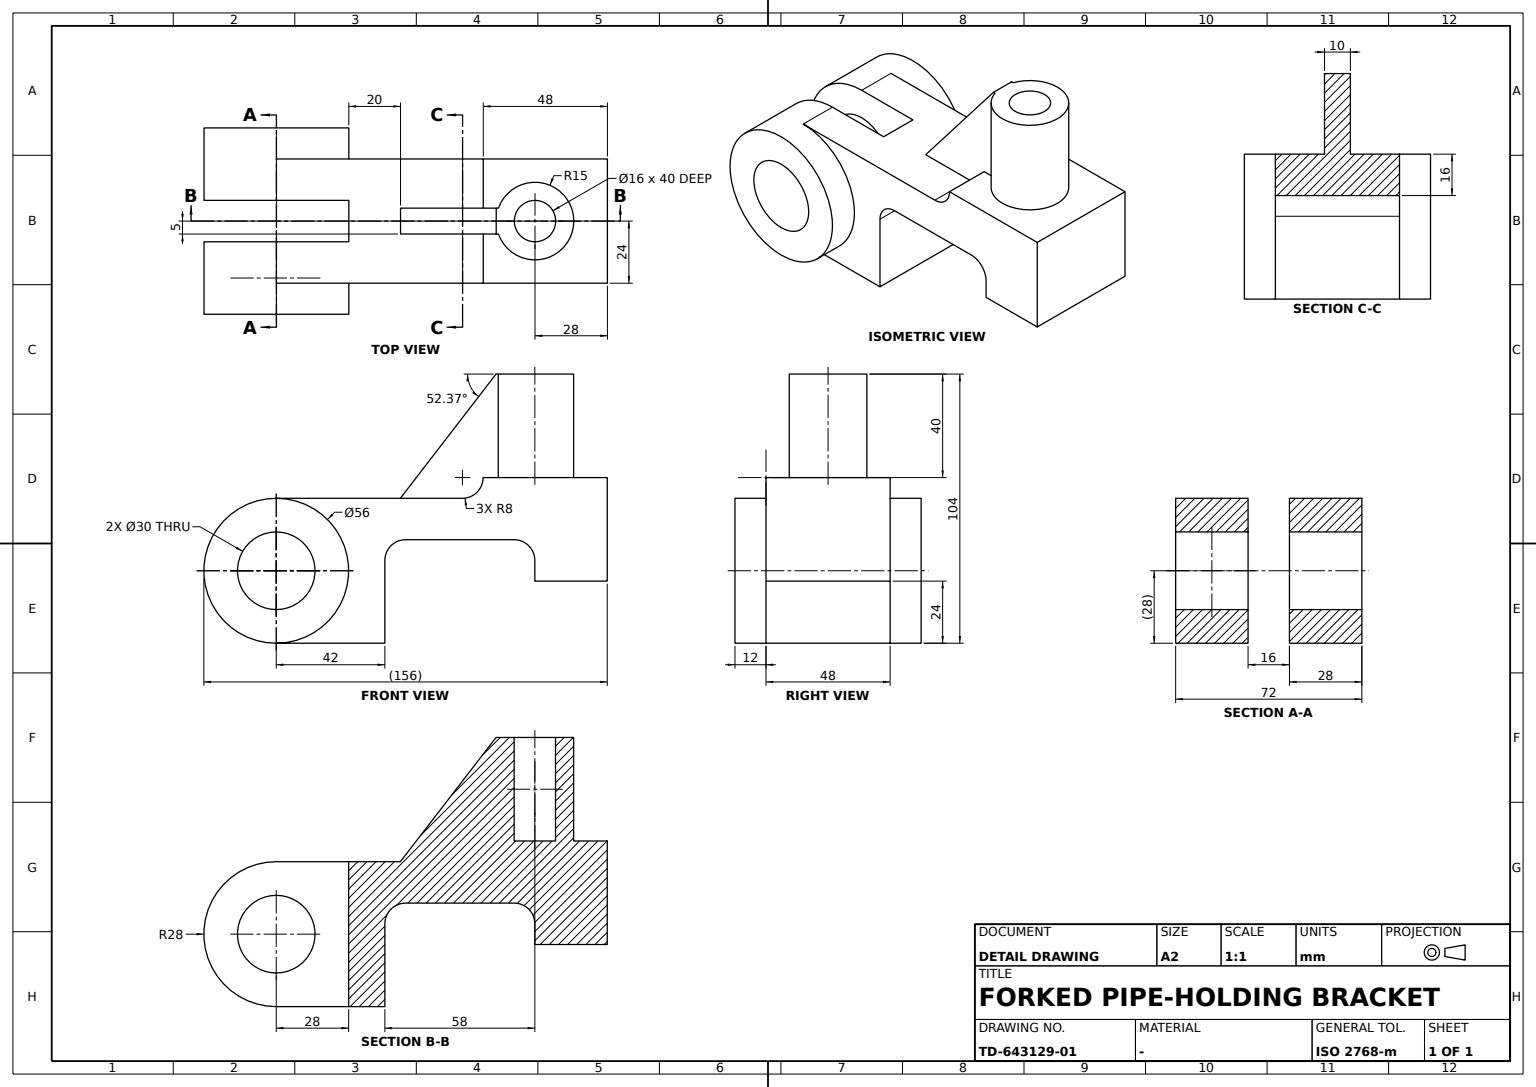
ISO-10303-21;
HEADER;
FILE_DESCRIPTION((''),'2;1');
FILE_NAME('','',(''),(''),'','','');
FILE_SCHEMA(('AUTOMOTIVE_DESIGN'));
ENDSEC;
DATA;
#1=APPLICATION_CONTEXT('');
#2=PRODUCT_CONTEXT('',#1,'mechanical');
#3=PRODUCT('','','',(#2));
#4=PRODUCT_DEFINITION_FORMATION('','',#3);
#5=PRODUCT_DEFINITION_CONTEXT('',#1,'design');
#6=PRODUCT_DEFINITION('','',#4,#5);
#7=PRODUCT_DEFINITION_SHAPE('','',#6);
#8=(LENGTH_UNIT()NAMED_UNIT(*)SI_UNIT(.MILLI.,.METRE.));
#9=(NAMED_UNIT(*)PLANE_ANGLE_UNIT()SI_UNIT($,.RADIAN.));
#10=(NAMED_UNIT(*)SI_UNIT($,.STERADIAN.)SOLID_ANGLE_UNIT());
#11=UNCERTAINTY_MEASURE_WITH_UNIT(LENGTH_MEASURE(0.005),#8,'distance_accuracy_value','');
#12=(GEOMETRIC_REPRESENTATION_CONTEXT(3)GLOBAL_UNCERTAINTY_ASSIGNED_CONTEXT((#11))GLOBAL_UNIT_ASSIGNED_CONTEXT((#8,#9,#10))REPRESENTATION_CONTEXT('',''));
#13=CARTESIAN_POINT('',(-24.,50.,12.));
#14=VERTEX_POINT('',#13);
#15=CARTESIAN_POINT('',(24.,50.,12.));
#16=VERTEX_POINT('',#15);
#17=CARTESIAN_POINT('',(0.,50.,12.));
#18=DIRECTION('',(1.,0.,0.));
#19=VECTOR('',#18,1000.);
#20=LINE('',#17,#19);
#21=EDGE_CURVE('',#14,#16,#20,.T.);
#22=ORIENTED_EDGE('',*,*,#21,.F.);
#23=CARTESIAN_POINT('',(-24.,92.,12.));
#24=VERTEX_POINT('',#23);
#25=CARTESIAN_POINT('',(-24.,0.,12.));
#26=DIRECTION('',(0.,-1.,0.));
#27=VECTOR('',#26,1000.);
#28=LINE('',#25,#27);
#29=EDGE_CURVE('',#24,#14,#28,.T.);
#30=ORIENTED_EDGE('',*,*,#29,.F.);
#31=CARTESIAN_POINT('',(24.,92.,12.));
#32=VERTEX_POINT('',#31);
#33=CARTESIAN_POINT('',(0.,92.,12.));
#34=LINE('',#33,#19);
#35=EDGE_CURVE('',#24,#32,#34,.T.);
#36=ORIENTED_EDGE('',*,*,#35,.T.);
#37=CARTESIAN_POINT('',(24.,0.,12.));
#38=LINE('',#37,#27);
#39=EDGE_CURVE('',#32,#16,#38,.T.);
#40=ORIENTED_EDGE('',*,*,#39,.T.);
#41=EDGE_LOOP('',(#22,#30,#36,#40));
#42=FACE_BOUND('',#41,.T.);
#43=DIRECTION('',(0.,0.,1.));
#44=AXIS2_PLACEMENT_3D('',#33,#43,#26);
#45=PLANE('',#44);
#46=ADVANCED_FACE('',(#42),#45,.F.);
#47=CARTESIAN_POINT('',(5.,85.857864,36.));
#48=VERTEX_POINT('',#47);
#49=CARTESIAN_POINT('',(5.,85.857864,76.));
#50=VERTEX_POINT('',#49);
#51=VECTOR('',#43,1000.);
#52=LINE('',#47,#51);
#53=EDGE_CURVE('',#48,#50,#52,.T.);
#54=ORIENTED_EDGE('',*,*,#53,.F.);
#55=CARTESIAN_POINT('',(-5.,85.857864,36.));
#56=VERTEX_POINT('',#55);
#57=CARTESIAN_POINT('',(0.,100.,36.));
#58=DIRECTION('',(0.,0.,-1.));
#59=DIRECTION('',(-1.,0.,0.));
#60=AXIS2_PLACEMENT_3D('',#57,#58,#59);
#61=CIRCLE('',#60,15.);
#62=EDGE_CURVE('',#48,#56,#61,.F.);
#63=ORIENTED_EDGE('',*,*,#62,.T.);
#64=CARTESIAN_POINT('',(-5.,85.857864,76.));
#65=VERTEX_POINT('',#64);
#66=LINE('',#55,#51);
#67=EDGE_CURVE('',#56,#65,#66,.T.);
#68=ORIENTED_EDGE('',*,*,#67,.T.);
#69=CARTESIAN_POINT('',(0.,100.,76.));
#70=AXIS2_PLACEMENT_3D('',#69,#43,#18);
#71=CIRCLE('',#70,15.);
#72=EDGE_CURVE('',#50,#65,#71,.T.);
#73=ORIENTED_EDGE('',*,*,#72,.F.);
#74=EDGE_LOOP('',(#54,#63,#68,#73));
#75=FACE_BOUND('',#74,.T.);
#76=CARTESIAN_POINT('',(0.,100.,56.));
#77=AXIS2_PLACEMENT_3D('',#76,#43,#18);
#78=CYLINDRICAL_SURFACE('',#77,15.);
#79=ADVANCED_FACE('',(#75),#78,.T.);
#80=CARTESIAN_POINT('',(-8.,28.,28.));
#81=VERTEX_POINT('',#80);
#82=CARTESIAN_POINT('',(-8.,28.,-28.));
#83=VERTEX_POINT('',#82);
#84=VECTOR('',#58,1000.);
#85=LINE('',#80,#84);
#86=EDGE_CURVE('',#81,#83,#85,.T.);
#87=ORIENTED_EDGE('',*,*,#86,.F.);
#88=CARTESIAN_POINT('',(-8.,0.,28.));
#89=VERTEX_POINT('',#88);
#90=LINE('',#88,#27);
#91=EDGE_CURVE('',#81,#89,#90,.T.);
#92=ORIENTED_EDGE('',*,*,#91,.T.);
#93=CARTESIAN_POINT('',(-8.,0.,-28.));
#94=VERTEX_POINT('',#93);
#95=CARTESIAN_POINT('',(-8.,0.,0.));
#96=AXIS2_PLACEMENT_3D('',#95,#18,#58);
#97=CIRCLE('',#96,28.);
#98=EDGE_CURVE('',#89,#94,#97,.T.);
#99=ORIENTED_EDGE('',*,*,#98,.T.);
#100=CARTESIAN_POINT('',(-8.,42.,-28.));
#101=DIRECTION('',(0.,1.,0.));
#102=VECTOR('',#101,1000.);
#103=LINE('',#100,#102);
#104=EDGE_CURVE('',#94,#83,#103,.T.);
#105=ORIENTED_EDGE('',*,*,#104,.T.);
#106=EDGE_LOOP('',(#87,#92,#99,#105));
#107=FACE_BOUND('',#106,.T.);
#108=CARTESIAN_POINT('',(-8.,0.,-15.));
#109=VERTEX_POINT('',#108);
#110=CIRCLE('',#96,15.);
#111=EDGE_CURVE('',#109,#109,#110,.T.);
#112=ORIENTED_EDGE('',*,*,#111,.F.);
#113=EDGE_LOOP('',(#112));
#114=FACE_BOUND('',#113,.T.);
#115=AXIS2_PLACEMENT_3D('',#80,#18,#26);
#116=PLANE('',#115);
#117=ADVANCED_FACE('',(#107,#114),#116,.T.);
#118=CARTESIAN_POINT('',(5.,72.,28.));
#119=VERTEX_POINT('',#118);
#120=CARTESIAN_POINT('',(5.,80.,36.));
#121=VERTEX_POINT('',#120);
#122=CARTESIAN_POINT('',(5.,72.,36.));
#123=AXIS2_PLACEMENT_3D('',#122,#18,#58);
#124=CIRCLE('',#123,8.);
#125=EDGE_CURVE('',#119,#121,#124,.T.);
#126=ORIENTED_EDGE('',*,*,#125,.F.);
#127=CARTESIAN_POINT('',(24.,72.,28.));
#128=VERTEX_POINT('',#127);
#129=CARTESIAN_POINT('',(0.,72.,28.));
#130=LINE('',#129,#19);
#131=EDGE_CURVE('',#119,#128,#130,.T.);
#132=ORIENTED_EDGE('',*,*,#131,.T.);
#133=CARTESIAN_POINT('',(24.,80.,36.));
#134=VERTEX_POINT('',#133);
#135=CARTESIAN_POINT('',(24.,72.,36.));
#136=AXIS2_PLACEMENT_3D('',#135,#18,#58);
#137=CIRCLE('',#136,8.);
#138=EDGE_CURVE('',#128,#134,#137,.T.);
#139=ORIENTED_EDGE('',*,*,#138,.T.);
#140=LINE('',#120,#19);
#141=EDGE_CURVE('',#121,#134,#140,.T.);
#142=ORIENTED_EDGE('',*,*,#141,.F.);
#143=EDGE_LOOP('',(#126,#132,#139,#142));
#144=FACE_BOUND('',#143,.T.);
#145=CARTESIAN_POINT('',(0.,72.,36.));
#146=AXIS2_PLACEMENT_3D('',#145,#18,#101);
#147=CYLINDRICAL_SURFACE('',#146,8.);
#148=ADVANCED_FACE('',(#144),#147,.F.);
#149=CARTESIAN_POINT('',(8.,0.,28.));
#150=VERTEX_POINT('',#149);
#151=CARTESIAN_POINT('',(8.,28.,28.));
#152=VERTEX_POINT('',#151);
#153=LINE('',#149,#102);
#154=EDGE_CURVE('',#150,#152,#153,.T.);
#155=ORIENTED_EDGE('',*,*,#154,.T.);
#156=CARTESIAN_POINT('',(8.,28.,-28.));
#157=VERTEX_POINT('',#156);
#158=LINE('',#151,#84);
#159=EDGE_CURVE('',#152,#157,#158,.T.);
#160=ORIENTED_EDGE('',*,*,#159,.T.);
#161=CARTESIAN_POINT('',(8.,0.,-28.));
#162=VERTEX_POINT('',#161);
#163=LINE('',#161,#102);
#164=EDGE_CURVE('',#162,#157,#163,.T.);
#165=ORIENTED_EDGE('',*,*,#164,.F.);
#166=CARTESIAN_POINT('',(8.,0.,0.));
#167=AXIS2_PLACEMENT_3D('',#166,#59,#43);
#168=CIRCLE('',#167,28.);
#169=EDGE_CURVE('',#150,#162,#168,.F.);
#170=ORIENTED_EDGE('',*,*,#169,.F.);
#171=EDGE_LOOP('',(#155,#160,#165,#170));
#172=FACE_BOUND('',#171,.T.);
#173=CARTESIAN_POINT('',(8.,0.,15.));
#174=VERTEX_POINT('',#173);
#175=CIRCLE('',#167,15.);
#176=EDGE_CURVE('',#174,#174,#175,.F.);
#177=ORIENTED_EDGE('',*,*,#176,.T.);
#178=EDGE_LOOP('',(#177));
#179=FACE_BOUND('',#178,.T.);
#180=AXIS2_PLACEMENT_3D('',#149,#59,#101);
#181=PLANE('',#180);
#182=ADVANCED_FACE('',(#172,#179),#181,.T.);
#183=CARTESIAN_POINT('',(-5.,48.,28.));
#184=VERTEX_POINT('',#183);
#185=CARTESIAN_POINT('',(-5.,72.,28.));
#186=VERTEX_POINT('',#185);
#187=CARTESIAN_POINT('',(-5.,0.,28.));
#188=LINE('',#187,#102);
#189=EDGE_CURVE('',#184,#186,#188,.T.);
#190=ORIENTED_EDGE('',*,*,#189,.F.);
#191=CARTESIAN_POINT('',(-5.,85.,76.));
#192=VERTEX_POINT('',#191);
#193=CARTESIAN_POINT('',(-5.,16.570651,-12.77321));
#194=DIRECTION('',(0.,-0.61050786,-0.792010197));
#195=VECTOR('',#194,1000.);
#196=LINE('',#193,#195);
#197=EDGE_CURVE('',#192,#184,#196,.T.);
#198=ORIENTED_EDGE('',*,*,#197,.F.);
#199=CARTESIAN_POINT('',(-5.,0.,76.));
#200=LINE('',#199,#102);
#201=EDGE_CURVE('',#192,#65,#200,.T.);
#202=ORIENTED_EDGE('',*,*,#201,.T.);
#203=ORIENTED_EDGE('',*,*,#67,.F.);
#204=CARTESIAN_POINT('',(-5.,80.,36.));
#205=VERTEX_POINT('',#204);
#206=CARTESIAN_POINT('',(-5.,0.,36.));
#207=LINE('',#206,#102);
#208=EDGE_CURVE('',#205,#56,#207,.T.);
#209=ORIENTED_EDGE('',*,*,#208,.F.);
#210=CARTESIAN_POINT('',(-5.,72.,36.));
#211=AXIS2_PLACEMENT_3D('',#210,#18,#58);
#212=CIRCLE('',#211,8.);
#213=EDGE_CURVE('',#186,#205,#212,.T.);
#214=ORIENTED_EDGE('',*,*,#213,.F.);
#215=EDGE_LOOP('',(#190,#198,#202,#203,#209,#214));
#216=FACE_BOUND('',#215,.T.);
#217=CARTESIAN_POINT('',(-5.,0.,0.));
#218=AXIS2_PLACEMENT_3D('',#217,#18,#101);
#219=PLANE('',#218);
#220=ADVANCED_FACE('',(#216),#219,.F.);
#221=LINE('',#82,#19);
#222=EDGE_CURVE('',#83,#157,#221,.T.);
#223=ORIENTED_EDGE('',*,*,#222,.F.);
#224=ORIENTED_EDGE('',*,*,#104,.F.);
#225=CARTESIAN_POINT('',(-24.,0.,-28.));
#226=VERTEX_POINT('',#225);
#227=CARTESIAN_POINT('',(-22.,0.,-28.));
#228=LINE('',#227,#19);
#229=EDGE_CURVE('',#226,#94,#228,.T.);
#230=ORIENTED_EDGE('',*,*,#229,.F.);
#231=CARTESIAN_POINT('',(-24.,42.,-28.));
#232=VERTEX_POINT('',#231);
#233=LINE('',#225,#27);
#234=EDGE_CURVE('',#232,#226,#233,.T.);
#235=ORIENTED_EDGE('',*,*,#234,.F.);
#236=CARTESIAN_POINT('',(24.,42.,-28.));
#237=VERTEX_POINT('',#236);
#238=CARTESIAN_POINT('',(0.,42.,-28.));
#239=LINE('',#238,#19);
#240=EDGE_CURVE('',#232,#237,#239,.T.);
#241=ORIENTED_EDGE('',*,*,#240,.T.);
#242=CARTESIAN_POINT('',(24.,0.,-28.));
#243=VERTEX_POINT('',#242);
#244=LINE('',#242,#27);
#245=EDGE_CURVE('',#237,#243,#244,.T.);
#246=ORIENTED_EDGE('',*,*,#245,.T.);
#247=EDGE_CURVE('',#162,#243,#228,.T.);
#248=ORIENTED_EDGE('',*,*,#247,.F.);
#249=ORIENTED_EDGE('',*,*,#164,.T.);
#250=EDGE_LOOP('',(#223,#224,#230,#235,#241,#246,#248,#249));
#251=FACE_BOUND('',#250,.T.);
#252=AXIS2_PLACEMENT_3D('',#238,#43,#26);
#253=PLANE('',#252);
#254=ADVANCED_FACE('',(#251),#253,.F.);
#255=CARTESIAN_POINT('',(5.,48.,28.));
#256=VERTEX_POINT('',#255);
#257=CARTESIAN_POINT('',(5.,0.,28.));
#258=LINE('',#257,#102);
#259=EDGE_CURVE('',#256,#119,#258,.T.);
#260=ORIENTED_EDGE('',*,*,#259,.T.);
#261=ORIENTED_EDGE('',*,*,#125,.T.);
#262=CARTESIAN_POINT('',(5.,0.,36.));
#263=LINE('',#262,#102);
#264=EDGE_CURVE('',#121,#48,#263,.T.);
#265=ORIENTED_EDGE('',*,*,#264,.T.);
#266=ORIENTED_EDGE('',*,*,#53,.T.);
#267=CARTESIAN_POINT('',(5.,85.,76.));
#268=VERTEX_POINT('',#267);
#269=CARTESIAN_POINT('',(5.,0.,76.));
#270=LINE('',#269,#102);
#271=EDGE_CURVE('',#268,#50,#270,.T.);
#272=ORIENTED_EDGE('',*,*,#271,.F.);
#273=CARTESIAN_POINT('',(5.,16.570651,-12.77321));
#274=LINE('',#273,#195);
#275=EDGE_CURVE('',#268,#256,#274,.T.);
#276=ORIENTED_EDGE('',*,*,#275,.T.);
#277=EDGE_LOOP('',(#260,#261,#265,#266,#272,#276));
#278=FACE_BOUND('',#277,.T.);
#279=CARTESIAN_POINT('',(5.,0.,0.));
#280=AXIS2_PLACEMENT_3D('',#279,#18,#101);
#281=PLANE('',#280);
#282=ADVANCED_FACE('',(#278),#281,.T.);
#283=CARTESIAN_POINT('',(-8.,100.,36.));
#284=VERTEX_POINT('',#283);
#285=CIRCLE('',#60,8.);
#286=EDGE_CURVE('',#284,#284,#285,.F.);
#287=ORIENTED_EDGE('',*,*,#286,.T.);
#288=EDGE_LOOP('',(#287));
#289=FACE_BOUND('',#288,.T.);
#290=CARTESIAN_POINT('',(0.,80.,36.));
#291=AXIS2_PLACEMENT_3D('',#290,#58,#101);
#292=PLANE('',#291);
#293=ADVANCED_FACE('',(#289),#292,.F.);
#294=CARTESIAN_POINT('',(-24.,128.,-4.));
#295=VERTEX_POINT('',#294);
#296=CARTESIAN_POINT('',(-24.,100.,-4.));
#297=VERTEX_POINT('',#296);
#298=CARTESIAN_POINT('',(-24.,0.,-4.));
#299=LINE('',#298,#27);
#300=EDGE_CURVE('',#295,#297,#299,.T.);
#301=ORIENTED_EDGE('',*,*,#300,.F.);
#302=CARTESIAN_POINT('',(24.,128.,-4.));
#303=VERTEX_POINT('',#302);
#304=CARTESIAN_POINT('',(0.,128.,-4.));
#305=LINE('',#304,#19);
#306=EDGE_CURVE('',#295,#303,#305,.T.);
#307=ORIENTED_EDGE('',*,*,#306,.T.);
#308=CARTESIAN_POINT('',(24.,100.,-4.));
#309=VERTEX_POINT('',#308);
#310=CARTESIAN_POINT('',(24.,0.,-4.));
#311=LINE('',#310,#27);
#312=EDGE_CURVE('',#303,#309,#311,.T.);
#313=ORIENTED_EDGE('',*,*,#312,.T.);
#314=CARTESIAN_POINT('',(0.,100.,-4.));
#315=LINE('',#314,#19);
#316=EDGE_CURVE('',#297,#309,#315,.T.);
#317=ORIENTED_EDGE('',*,*,#316,.F.);
#318=EDGE_LOOP('',(#301,#307,#313,#317));
#319=FACE_BOUND('',#318,.T.);
#320=AXIS2_PLACEMENT_3D('',#304,#43,#26);
#321=PLANE('',#320);
#322=ADVANCED_FACE('',(#319),#321,.F.);
#323=ORIENTED_EDGE('',*,*,#35,.F.);
#324=CARTESIAN_POINT('',(-24.,100.,4.));
#325=VERTEX_POINT('',#324);
#326=CARTESIAN_POINT('',(-24.,92.,4.));
#327=AXIS2_PLACEMENT_3D('',#326,#18,#58);
#328=CIRCLE('',#327,8.);
#329=EDGE_CURVE('',#325,#24,#328,.T.);
#330=ORIENTED_EDGE('',*,*,#329,.F.);
#331=CARTESIAN_POINT('',(24.,100.,4.));
#332=VERTEX_POINT('',#331);
#333=CARTESIAN_POINT('',(0.,100.,4.));
#334=LINE('',#333,#19);
#335=EDGE_CURVE('',#325,#332,#334,.T.);
#336=ORIENTED_EDGE('',*,*,#335,.T.);
#337=CARTESIAN_POINT('',(24.,92.,4.));
#338=AXIS2_PLACEMENT_3D('',#337,#18,#58);
#339=CIRCLE('',#338,8.);
#340=EDGE_CURVE('',#332,#32,#339,.T.);
#341=ORIENTED_EDGE('',*,*,#340,.T.);
#342=EDGE_LOOP('',(#323,#330,#336,#341));
#343=FACE_BOUND('',#342,.T.);
#344=CARTESIAN_POINT('',(0.,92.,4.));
#345=AXIS2_PLACEMENT_3D('',#344,#18,#101);
#346=CYLINDRICAL_SURFACE('',#345,8.);
#347=ADVANCED_FACE('',(#343),#346,.F.);
#348=CARTESIAN_POINT('',(36.,0.,-28.));
#349=VERTEX_POINT('',#348);
#350=CARTESIAN_POINT('',(36.,0.,0.));
#351=AXIS2_PLACEMENT_3D('',#350,#18,#58);
#352=CIRCLE('',#351,28.);
#353=EDGE_CURVE('',#349,#349,#352,.T.);
#354=ORIENTED_EDGE('',*,*,#353,.F.);
#355=EDGE_LOOP('',(#354));
#356=FACE_BOUND('',#355,.T.);
#357=ORIENTED_EDGE('',*,*,#247,.T.);
#358=CARTESIAN_POINT('',(24.,0.,28.));
#359=VERTEX_POINT('',#358);
#360=CARTESIAN_POINT('',(24.,0.,0.));
#361=AXIS2_PLACEMENT_3D('',#360,#18,#58);
#362=CIRCLE('',#361,28.);
#363=EDGE_CURVE('',#243,#359,#362,.T.);
#364=ORIENTED_EDGE('',*,*,#363,.T.);
#365=CARTESIAN_POINT('',(-22.,0.,28.));
#366=LINE('',#365,#19);
#367=EDGE_CURVE('',#150,#359,#366,.T.);
#368=ORIENTED_EDGE('',*,*,#367,.F.);
#369=ORIENTED_EDGE('',*,*,#169,.T.);
#370=EDGE_LOOP('',(#357,#364,#368,#369));
#371=FACE_BOUND('',#370,.T.);
#372=CARTESIAN_POINT('',(-22.,0.,0.));
#373=AXIS2_PLACEMENT_3D('',#372,#18,#101);
#374=CYLINDRICAL_SURFACE('',#373,28.);
#375=ADVANCED_FACE('',(#356,#371),#374,.T.);
#376=CARTESIAN_POINT('',(24.,42.,4.));
#377=VERTEX_POINT('',#376);
#378=CARTESIAN_POINT('',(24.,42.,0.));
#379=LINE('',#378,#84);
#380=EDGE_CURVE('',#377,#237,#379,.T.);
#381=ORIENTED_EDGE('',*,*,#380,.T.);
#382=ORIENTED_EDGE('',*,*,#240,.F.);
#383=CARTESIAN_POINT('',(-24.,42.,4.));
#384=VERTEX_POINT('',#383);
#385=CARTESIAN_POINT('',(-24.,42.,0.));
#386=LINE('',#385,#84);
#387=EDGE_CURVE('',#384,#232,#386,.T.);
#388=ORIENTED_EDGE('',*,*,#387,.F.);
#389=CARTESIAN_POINT('',(0.,42.,4.));
#390=LINE('',#389,#19);
#391=EDGE_CURVE('',#384,#377,#390,.T.);
#392=ORIENTED_EDGE('',*,*,#391,.T.);
#393=EDGE_LOOP('',(#381,#382,#388,#392));
#394=FACE_BOUND('',#393,.T.);
#395=AXIS2_PLACEMENT_3D('',#389,#26,#58);
#396=PLANE('',#395);
#397=ADVANCED_FACE('',(#394),#396,.F.);
#398=CARTESIAN_POINT('',(-24.,128.,36.));
#399=VERTEX_POINT('',#398);
#400=CARTESIAN_POINT('',(24.,128.,36.));
#401=VERTEX_POINT('',#400);
#402=CARTESIAN_POINT('',(0.,128.,36.));
#403=LINE('',#402,#19);
#404=EDGE_CURVE('',#399,#401,#403,.T.);
#405=ORIENTED_EDGE('',*,*,#404,.T.);
#406=CARTESIAN_POINT('',(24.,128.,0.));
#407=LINE('',#406,#84);
#408=EDGE_CURVE('',#401,#303,#407,.T.);
#409=ORIENTED_EDGE('',*,*,#408,.T.);
#410=ORIENTED_EDGE('',*,*,#306,.F.);
#411=CARTESIAN_POINT('',(-24.,128.,0.));
#412=LINE('',#411,#84);
#413=EDGE_CURVE('',#399,#295,#412,.T.);
#414=ORIENTED_EDGE('',*,*,#413,.F.);
#415=EDGE_LOOP('',(#405,#409,#410,#414));
#416=FACE_BOUND('',#415,.T.);
#417=AXIS2_PLACEMENT_3D('',#402,#26,#58);
#418=PLANE('',#417);
#419=ADVANCED_FACE('',(#416),#418,.F.);
#420=ORIENTED_EDGE('',*,*,#98,.F.);
#421=CARTESIAN_POINT('',(-24.,0.,28.));
#422=VERTEX_POINT('',#421);
#423=EDGE_CURVE('',#422,#89,#366,.T.);
#424=ORIENTED_EDGE('',*,*,#423,.F.);
#425=CARTESIAN_POINT('',(-24.,0.,0.));
#426=AXIS2_PLACEMENT_3D('',#425,#18,#58);
#427=CIRCLE('',#426,28.);
#428=EDGE_CURVE('',#226,#422,#427,.T.);
#429=ORIENTED_EDGE('',*,*,#428,.F.);
#430=ORIENTED_EDGE('',*,*,#229,.T.);
#431=EDGE_LOOP('',(#420,#424,#429,#430));
#432=FACE_BOUND('',#431,.T.);
#433=CARTESIAN_POINT('',(-36.,0.,-28.));
#434=VERTEX_POINT('',#433);
#435=CARTESIAN_POINT('',(-36.,0.,0.));
#436=AXIS2_PLACEMENT_3D('',#435,#18,#58);
#437=CIRCLE('',#436,28.);
#438=EDGE_CURVE('',#434,#434,#437,.T.);
#439=ORIENTED_EDGE('',*,*,#438,.T.);
#440=EDGE_LOOP('',(#439));
#441=FACE_BOUND('',#440,.T.);
#442=ADVANCED_FACE('',(#432,#441),#374,.T.);
#443=CARTESIAN_POINT('',(0.,28.,28.));
#444=LINE('',#443,#19);
#445=EDGE_CURVE('',#81,#152,#444,.T.);
#446=ORIENTED_EDGE('',*,*,#445,.T.);
#447=ORIENTED_EDGE('',*,*,#154,.F.);
#448=ORIENTED_EDGE('',*,*,#367,.T.);
#449=LINE('',#358,#102);
#450=EDGE_CURVE('',#359,#128,#449,.T.);
#451=ORIENTED_EDGE('',*,*,#450,.T.);
#452=ORIENTED_EDGE('',*,*,#131,.F.);
#453=ORIENTED_EDGE('',*,*,#259,.F.);
#454=CARTESIAN_POINT('',(0.,48.,28.));
#455=LINE('',#454,#19);
#456=EDGE_CURVE('',#184,#256,#455,.T.);
#457=ORIENTED_EDGE('',*,*,#456,.F.);
#458=ORIENTED_EDGE('',*,*,#189,.T.);
#459=CARTESIAN_POINT('',(-24.,72.,28.));
#460=VERTEX_POINT('',#459);
#461=EDGE_CURVE('',#460,#186,#130,.T.);
#462=ORIENTED_EDGE('',*,*,#461,.F.);
#463=LINE('',#421,#102);
#464=EDGE_CURVE('',#422,#460,#463,.T.);
#465=ORIENTED_EDGE('',*,*,#464,.F.);
#466=ORIENTED_EDGE('',*,*,#423,.T.);
#467=ORIENTED_EDGE('',*,*,#91,.F.);
#468=EDGE_LOOP('',(#446,#447,#448,#451,#452,#453,#457,#458,#462,#465,#466,#467));
#469=FACE_BOUND('',#468,.T.);
#470=CARTESIAN_POINT('',(0.,0.,28.));
#471=AXIS2_PLACEMENT_3D('',#470,#58,#101);
#472=PLANE('',#471);
#473=ADVANCED_FACE('',(#469),#472,.F.);
#474=ORIENTED_EDGE('',*,*,#197,.T.);
#475=ORIENTED_EDGE('',*,*,#456,.T.);
#476=ORIENTED_EDGE('',*,*,#275,.F.);
#477=CARTESIAN_POINT('',(0.,85.,76.));
#478=LINE('',#477,#19);
#479=EDGE_CURVE('',#192,#268,#478,.T.);
#480=ORIENTED_EDGE('',*,*,#479,.F.);
#481=EDGE_LOOP('',(#474,#475,#476,#480));
#482=FACE_BOUND('',#481,.T.);
#483=DIRECTION('',(0.,-0.792010197,0.61050786));
#484=AXIS2_PLACEMENT_3D('',#477,#483,#194);
#485=PLANE('',#484);
#486=ADVANCED_FACE('',(#482),#485,.T.);
#487=ORIENTED_EDGE('',*,*,#479,.T.);
#488=ORIENTED_EDGE('',*,*,#271,.T.);
#489=ORIENTED_EDGE('',*,*,#72,.T.);
#490=ORIENTED_EDGE('',*,*,#201,.F.);
#491=EDGE_LOOP('',(#487,#488,#489,#490));
#492=FACE_BOUND('',#491,.T.);
#493=CARTESIAN_POINT('',(8.,100.,76.));
#494=VERTEX_POINT('',#493);
#495=CIRCLE('',#70,8.);
#496=EDGE_CURVE('',#494,#494,#495,.T.);
#497=ORIENTED_EDGE('',*,*,#496,.F.);
#498=EDGE_LOOP('',(#497));
#499=FACE_BOUND('',#498,.T.);
#500=CARTESIAN_POINT('',(0.,0.,76.));
#501=AXIS2_PLACEMENT_3D('',#500,#43,#18);
#502=PLANE('',#501);
#503=ADVANCED_FACE('',(#492,#499),#502,.T.);
#504=ORIENTED_EDGE('',*,*,#413,.T.);
#505=ORIENTED_EDGE('',*,*,#300,.T.);
#506=CARTESIAN_POINT('',(-24.,100.,0.));
#507=LINE('',#506,#51);
#508=EDGE_CURVE('',#297,#325,#507,.T.);
#509=ORIENTED_EDGE('',*,*,#508,.T.);
#510=ORIENTED_EDGE('',*,*,#329,.T.);
#511=ORIENTED_EDGE('',*,*,#29,.T.);
#512=CARTESIAN_POINT('',(-24.,50.,4.));
#513=AXIS2_PLACEMENT_3D('',#512,#18,#58);
#514=CIRCLE('',#513,8.);
#515=EDGE_CURVE('',#14,#384,#514,.T.);
#516=ORIENTED_EDGE('',*,*,#515,.T.);
#517=ORIENTED_EDGE('',*,*,#387,.T.);
#518=ORIENTED_EDGE('',*,*,#234,.T.);
#519=ORIENTED_EDGE('',*,*,#428,.T.);
#520=ORIENTED_EDGE('',*,*,#464,.T.);
#521=CARTESIAN_POINT('',(-24.,80.,36.));
#522=VERTEX_POINT('',#521);
#523=CARTESIAN_POINT('',(-24.,72.,36.));
#524=AXIS2_PLACEMENT_3D('',#523,#18,#58);
#525=CIRCLE('',#524,8.);
#526=EDGE_CURVE('',#460,#522,#525,.T.);
#527=ORIENTED_EDGE('',*,*,#526,.T.);
#528=CARTESIAN_POINT('',(-24.,0.,36.));
#529=LINE('',#528,#102);
#530=EDGE_CURVE('',#522,#399,#529,.T.);
#531=ORIENTED_EDGE('',*,*,#530,.T.);
#532=EDGE_LOOP('',(#504,#505,#509,#510,#511,#516,#517,#518,#519,#520,#527,#531));
#533=FACE_BOUND('',#532,.T.);
#534=AXIS2_PLACEMENT_3D('',#425,#18,#101);
#535=PLANE('',#534);
#536=ADVANCED_FACE('',(#533),#535,.F.);
#537=ORIENTED_EDGE('',*,*,#111,.T.);
#538=EDGE_LOOP('',(#537));
#539=FACE_BOUND('',#538,.T.);
#540=CARTESIAN_POINT('',(-36.,0.,-15.));
#541=VERTEX_POINT('',#540);
#542=CIRCLE('',#436,15.);
#543=EDGE_CURVE('',#541,#541,#542,.T.);
#544=ORIENTED_EDGE('',*,*,#543,.F.);
#545=EDGE_LOOP('',(#544));
#546=FACE_BOUND('',#545,.T.);
#547=CYLINDRICAL_SURFACE('',#373,15.);
#548=ADVANCED_FACE('',(#539,#546),#547,.F.);
#549=LINE('',#521,#19);
#550=EDGE_CURVE('',#522,#205,#549,.T.);
#551=ORIENTED_EDGE('',*,*,#550,.F.);
#552=ORIENTED_EDGE('',*,*,#526,.F.);
#553=ORIENTED_EDGE('',*,*,#461,.T.);
#554=ORIENTED_EDGE('',*,*,#213,.T.);
#555=EDGE_LOOP('',(#551,#552,#553,#554));
#556=FACE_BOUND('',#555,.T.);
#557=ADVANCED_FACE('',(#556),#147,.F.);
#558=ORIENTED_EDGE('',*,*,#445,.F.);
#559=ORIENTED_EDGE('',*,*,#86,.T.);
#560=ORIENTED_EDGE('',*,*,#222,.T.);
#561=ORIENTED_EDGE('',*,*,#159,.F.);
#562=EDGE_LOOP('',(#558,#559,#560,#561));
#563=FACE_BOUND('',#562,.T.);
#564=AXIS2_PLACEMENT_3D('',#80,#101,#18);
#565=PLANE('',#564);
#566=ADVANCED_FACE('',(#563),#565,.F.);
#567=ORIENTED_EDGE('',*,*,#286,.F.);
#568=EDGE_LOOP('',(#567));
#569=FACE_BOUND('',#568,.T.);
#570=ORIENTED_EDGE('',*,*,#496,.T.);
#571=EDGE_LOOP('',(#570));
#572=FACE_BOUND('',#571,.T.);
#573=CYLINDRICAL_SURFACE('',#77,8.);
#574=ADVANCED_FACE('',(#569,#572),#573,.F.);
#575=ORIENTED_EDGE('',*,*,#353,.T.);
#576=EDGE_LOOP('',(#575));
#577=FACE_BOUND('',#576,.T.);
#578=CARTESIAN_POINT('',(36.,0.,-15.));
#579=VERTEX_POINT('',#578);
#580=CIRCLE('',#351,15.);
#581=EDGE_CURVE('',#579,#579,#580,.T.);
#582=ORIENTED_EDGE('',*,*,#581,.F.);
#583=EDGE_LOOP('',(#582));
#584=FACE_BOUND('',#583,.T.);
#585=AXIS2_PLACEMENT_3D('',#350,#18,#101);
#586=PLANE('',#585);
#587=ADVANCED_FACE('',(#577,#584),#586,.T.);
#588=ORIENTED_EDGE('',*,*,#176,.F.);
#589=EDGE_LOOP('',(#588));
#590=FACE_BOUND('',#589,.T.);
#591=ORIENTED_EDGE('',*,*,#581,.T.);
#592=EDGE_LOOP('',(#591));
#593=FACE_BOUND('',#592,.T.);
#594=ADVANCED_FACE('',(#590,#593),#547,.F.);
#595=ORIENTED_EDGE('',*,*,#312,.F.);
#596=ORIENTED_EDGE('',*,*,#408,.F.);
#597=CARTESIAN_POINT('',(24.,0.,36.));
#598=LINE('',#597,#102);
#599=EDGE_CURVE('',#134,#401,#598,.T.);
#600=ORIENTED_EDGE('',*,*,#599,.F.);
#601=ORIENTED_EDGE('',*,*,#138,.F.);
#602=ORIENTED_EDGE('',*,*,#450,.F.);
#603=ORIENTED_EDGE('',*,*,#363,.F.);
#604=ORIENTED_EDGE('',*,*,#245,.F.);
#605=ORIENTED_EDGE('',*,*,#380,.F.);
#606=CARTESIAN_POINT('',(24.,50.,4.));
#607=AXIS2_PLACEMENT_3D('',#606,#18,#58);
#608=CIRCLE('',#607,8.);
#609=EDGE_CURVE('',#16,#377,#608,.T.);
#610=ORIENTED_EDGE('',*,*,#609,.F.);
#611=ORIENTED_EDGE('',*,*,#39,.F.);
#612=ORIENTED_EDGE('',*,*,#340,.F.);
#613=CARTESIAN_POINT('',(24.,100.,0.));
#614=LINE('',#613,#51);
#615=EDGE_CURVE('',#309,#332,#614,.T.);
#616=ORIENTED_EDGE('',*,*,#615,.F.);
#617=EDGE_LOOP('',(#595,#596,#600,#601,#602,#603,#604,#605,#610,#611,#612,#616));
#618=FACE_BOUND('',#617,.T.);
#619=AXIS2_PLACEMENT_3D('',#360,#18,#101);
#620=PLANE('',#619);
#621=ADVANCED_FACE('',(#618),#620,.T.);
#622=ORIENTED_EDGE('',*,*,#62,.F.);
#623=ORIENTED_EDGE('',*,*,#264,.F.);
#624=ORIENTED_EDGE('',*,*,#141,.T.);
#625=ORIENTED_EDGE('',*,*,#599,.T.);
#626=ORIENTED_EDGE('',*,*,#404,.F.);
#627=ORIENTED_EDGE('',*,*,#530,.F.);
#628=ORIENTED_EDGE('',*,*,#550,.T.);
#629=ORIENTED_EDGE('',*,*,#208,.T.);
#630=EDGE_LOOP('',(#622,#623,#624,#625,#626,#627,#628,#629));
#631=FACE_BOUND('',#630,.T.);
#632=ADVANCED_FACE('',(#631),#292,.F.);
#633=ORIENTED_EDGE('',*,*,#615,.T.);
#634=ORIENTED_EDGE('',*,*,#335,.F.);
#635=ORIENTED_EDGE('',*,*,#508,.F.);
#636=ORIENTED_EDGE('',*,*,#316,.T.);
#637=EDGE_LOOP('',(#633,#634,#635,#636));
#638=FACE_BOUND('',#637,.T.);
#639=AXIS2_PLACEMENT_3D('',#314,#101,#43);
#640=PLANE('',#639);
#641=ADVANCED_FACE('',(#638),#640,.F.);
#642=ORIENTED_EDGE('',*,*,#515,.F.);
#643=ORIENTED_EDGE('',*,*,#21,.T.);
#644=ORIENTED_EDGE('',*,*,#609,.T.);
#645=ORIENTED_EDGE('',*,*,#391,.F.);
#646=EDGE_LOOP('',(#642,#643,#644,#645));
#647=FACE_BOUND('',#646,.T.);
#648=CARTESIAN_POINT('',(0.,50.,4.));
#649=AXIS2_PLACEMENT_3D('',#648,#18,#101);
#650=CYLINDRICAL_SURFACE('',#649,8.);
#651=ADVANCED_FACE('',(#647),#650,.F.);
#652=ORIENTED_EDGE('',*,*,#438,.F.);
#653=EDGE_LOOP('',(#652));
#654=FACE_BOUND('',#653,.T.);
#655=ORIENTED_EDGE('',*,*,#543,.T.);
#656=EDGE_LOOP('',(#655));
#657=FACE_BOUND('',#656,.T.);
#658=AXIS2_PLACEMENT_3D('',#435,#18,#101);
#659=PLANE('',#658);
#660=ADVANCED_FACE('',(#654,#657),#659,.F.);
#661=CLOSED_SHELL('',(#46,#79,#117,#148,#182,#220,#254,#282,#293,#322,#347,#375,#397,#419,#442,#473,#486,#503,#536,#548,#557,#566,#574,#587,#594,#621,#632,#641,#651,#660));
#662=MANIFOLD_SOLID_BREP('',#661);
#663=ADVANCED_BREP_SHAPE_REPRESENTATION('',(#662),#12);
#664=SHAPE_DEFINITION_REPRESENTATION(#7,#663);
ENDSEC;
END-ISO-10303-21;
